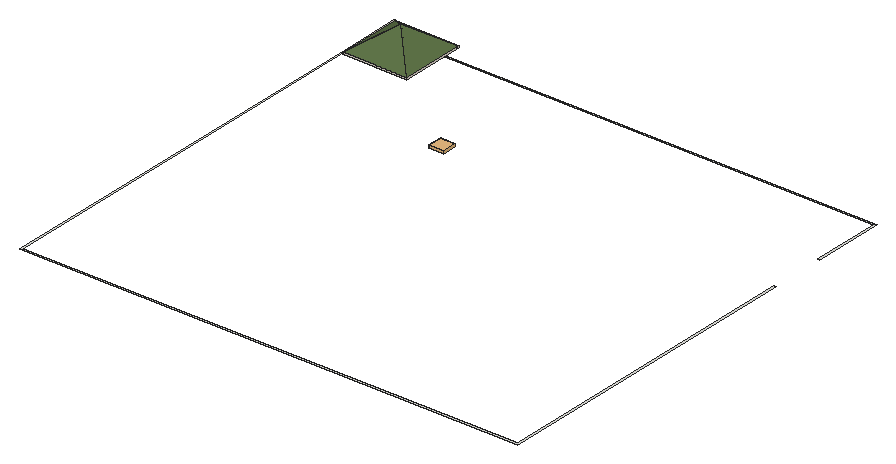
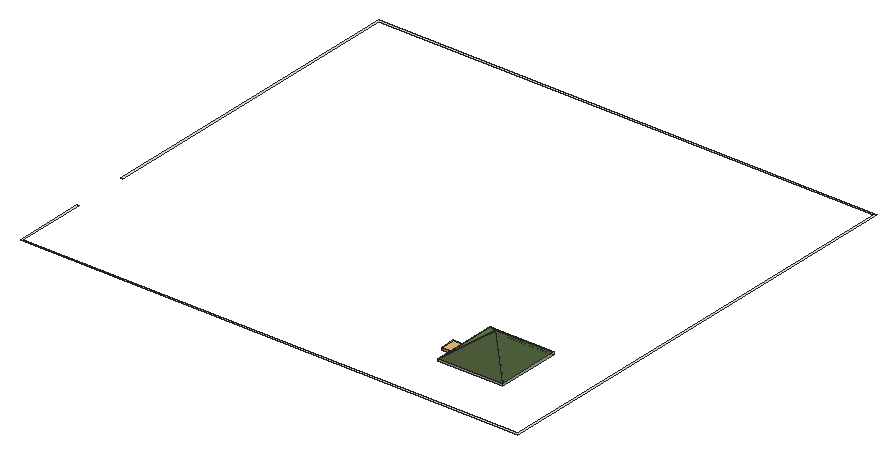
# SketchUp Ruby script. Lengths in inches.
U = 1.inch
M = Sketchup.active_model
def pt(a) = Geom::Point3d.new(a.map { |v| v * U })
def face(e, loops, mat)
  f = e.add_face(loops[0].map { |a| pt(a) })
  loops[1..].each { |l| e.add_face(l.map { |a| pt(a) }).erase! }
  f.material = f.back_material = mat if mat
  f
end
# faces: each face lists its corners as indices into pts; further lists are holes
def faces(e, pts, list, mat = nil) = list.each { |f| face(e, (f[0].is_a?(Array) ? f : [f]).map { |l| l.map { |i| pts[i] } }, mat) }
# xy, xz, yz: faces in a plane at the given z, y or x. An outline is a flat list of corners, or four numbers for a rectangle; further outlines are holes
def ring(l) = l.size == 4 ? [[l[0], l[1]], [l[2], l[1]], [l[2], l[3]], [l[0], l[3]]] : l.each_slice(2).to_a
def flat(e, list, mat, &to3) = list.each { |f| face(e, (f[0].is_a?(Array) ? f : [f]).map { |l| ring(l).map { |u, v| to3.(u, v) } }, mat) }
def xy(e, z, list, mat = nil) = flat(e, list, mat) { |x, y| [x, y, z] }
def xz(e, y, list, mat = nil) = flat(e, list, mat) { |x, z| [x, y, z] }
def yz(e, x, list, mat = nil) = flat(e, list, mat) { |y, z| [x, y, z] }
def lines(e, pts, list) = list.each { |a, b| e.add_line(pt(pts[a]), pt(pts[b])) }
# prism: a flat outline (further loops are holes) pulled along v
def prism(e, loops, v, mat = nil)
  f = face(e, loops, mat); d = Geom::Vector3d.new(v.map { |x| x * U })
  f.pushpull(f.normal.samedirection?(d) ? d.length : -d.length)
end
def box(e, o, s, mat = nil) = prism(e, [[o, [o[0] + s[0], o[1], o[2]], [o[0] + s[0], o[1] + s[1], o[2]], [o[0], o[1] + s[1], o[2]]]], [0, 0, s[2]], mat)
def at(x, y, z, deg = 0) = Geom::Transformation.translation(pt([x, y, z])) * Geom::Transformation.rotation(ORIGIN, Z_AXIS, deg.degrees)
def axes(o, x, y, z) = Geom::Transformation.new([*x, 0, *y, 0, *z, 0, *pt(o).to_a, 1])
def part(name) = M.definitions.add(name)
# library, detail: a bought-in or finely detailed component or shape, given as its bounding box
def library(name, o, s) = part(name).tap { |d| box(d.entities, o, s) }
def detail(e, o, s) = box(e.add_group.entities, o, s)
def put(e, d, t, mat = nil) = e.add_instance(d, t).tap { |i| i.material = mat if mat }
def group(e, t, mat = nil) = e.add_group.tap { |g| g.transformation = t; g.material = mat if mat }.entities
root = M.entities
M.materials.add("Marble_01_1K").color = [230, 221, 211]
M.materials.add("Material__1").color = [95, 70, 46]
M.materials.add("Roofing_01_1K").color = [84, 79, 73]
M.materials.add("Roofing_02_1K").color = [97, 118, 74]
c1 = library("Group\#17",[-876.58,-99.29,706.19],[35.74,35.58,5.93])
c2 = part("Group199\#1")
xz(c2.entities,880.3,[[72.19,120,228.37,125]],"Marble_01_1K")
xz(c2.entities,1036.47,[[72.19,120,228.37,125]],"Marble_01_1K")
yz(c2.entities,72.19,[[880.3,120,1036.47,125]],"Marble_01_1K")
yz(c2.entities,228.37,[[880.3,120,1036.47,125]],"Marble_01_1K")
p = [[228.37,880.3,120],[150.28,958.39,174.68],[72.19,880.3,120],[72.19,1036.47,120],[228.37,880.3,125],[150.28,958.39,179.68],
  [72.19,1036.47,125],[228.37,1036.47,120],[228.37,1036.47,125],[72.19,880.3,125]]
faces(c2.entities,p,[[0,1,2],[2,1,3],[0,4,5,6,3,1],[7,8,5,9,2,1],[7,1,0],[3,1,7]])
faces(c2.entities,p,[[4,5,9],[9,5,6],[8,5,4],[6,5,8]],"Roofing_02_1K")
c3 = part("Group198\#1")
p = [[228.37,880.3,120],[72.19,880.3,120],[72.19,1036.47,120],[228.37,1036.47,120]]
lines(c3.entities,p,[[0,1],[2,3],[1,2],[3,0]])
put(c3.entities,c2,at(0,0,0),"Roofing_01_1K")
xy(root,60,[[8.46,0.95,1208.46,0.95,1208.46,777.17,1204.46,777.17,1204.46,4.95,12.46,4.95,12.46,1076.74,1204.46,1076.74,1204.46,910.21,1208.46,910.21,1208.46,1080.74,8.46,1080.74]])
put(root,c1,at(1203.01,933.0625,-680.87),"Material__1")
put(root,c3,at(8.46,0.95,0))
